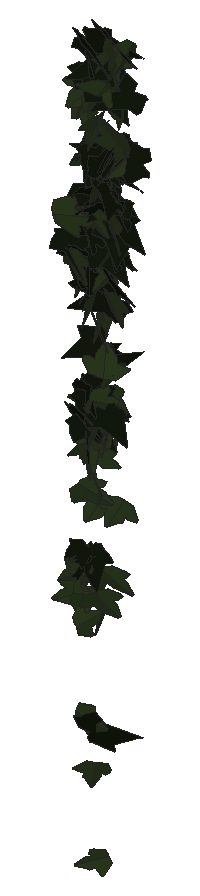
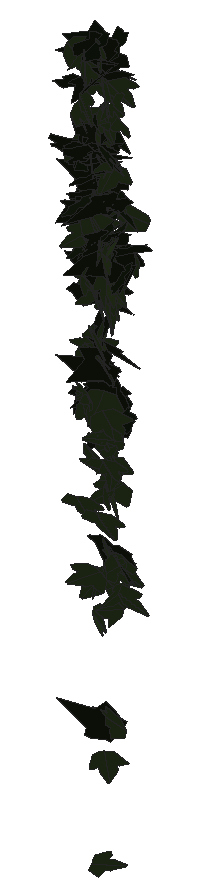
# SketchUp Ruby script. Lengths in inches.
U = 1.inch
M = Sketchup.active_model
def pt(a) = Geom::Point3d.new(a.map { |v| v * U })
def face(e, loops, mat)
  f = e.add_face(loops[0].map { |a| pt(a) })
  loops[1..].each { |l| e.add_face(l.map { |a| pt(a) }).erase! }
  f.material = f.back_material = mat if mat
  f
end
# faces: each face lists its corners as indices into pts; further lists are holes
def faces(e, pts, list, mat = nil) = list.each { |f| face(e, (f[0].is_a?(Array) ? f : [f]).map { |l| l.map { |i| pts[i] } }, mat) }
# xy, xz, yz: faces in a plane at the given z, y or x. An outline is a flat list of corners, or four numbers for a rectangle; further outlines are holes
def ring(l) = l.size == 4 ? [[l[0], l[1]], [l[2], l[1]], [l[2], l[3]], [l[0], l[3]]] : l.each_slice(2).to_a
def flat(e, list, mat, &to3) = list.each { |f| face(e, (f[0].is_a?(Array) ? f : [f]).map { |l| ring(l).map { |u, v| to3.(u, v) } }, mat) }
def xy(e, z, list, mat = nil) = flat(e, list, mat) { |x, y| [x, y, z] }
def xz(e, y, list, mat = nil) = flat(e, list, mat) { |x, z| [x, y, z] }
def yz(e, x, list, mat = nil) = flat(e, list, mat) { |y, z| [x, y, z] }
def lines(e, pts, list) = list.each { |a, b| e.add_line(pt(pts[a]), pt(pts[b])) }
# prism: a flat outline (further loops are holes) pulled along v
def prism(e, loops, v, mat = nil)
  f = face(e, loops, mat); d = Geom::Vector3d.new(v.map { |x| x * U })
  f.pushpull(f.normal.samedirection?(d) ? d.length : -d.length)
end
def box(e, o, s, mat = nil) = prism(e, [[o, [o[0] + s[0], o[1], o[2]], [o[0] + s[0], o[1] + s[1], o[2]], [o[0], o[1] + s[1], o[2]]]], [0, 0, s[2]], mat)
def at(x, y, z, deg = 0) = Geom::Transformation.translation(pt([x, y, z])) * Geom::Transformation.rotation(ORIGIN, Z_AXIS, deg.degrees)
def axes(o, x, y, z) = Geom::Transformation.new([*x, 0, *y, 0, *z, 0, *pt(o).to_a, 1])
def part(name) = M.definitions.add(name)
# library, detail: a bought-in or finely detailed component or shape, given as its bounding box
def library(name, o, s) = part(name).tap { |d| box(d.entities, o, s) }
def detail(e, o, s) = box(e.add_group.entities, o, s)
def put(e, d, t, mat = nil) = e.add_instance(d, t).tap { |i| i.material = mat if mat }
def group(e, t, mat = nil) = e.add_group.tap { |g| g.transformation = t; g.material = mat if mat }.entities
root = M.entities
M.materials.add("1026 AP 7946 SUNNY SIDE UP").color = [254, 231, 186]
M.materials.add("efeu1").color = [18, 25, 13]
M.materials.add("efeu2").color = [43, 57, 29]
c1 = part("ivyleaf_10")
p = [[0,0.5,-0.03],[-0.0625,2.02,-0.43],[-0.19,2.01,-0.46],[-0.54,1.05,-0.29],[-0.52,0.625,-0.18],[-0.83,0.76,-0.28],
  [-1.16,0.64,-0.33],[-1.15,0.33,-0.24],[-0.77,-0.39,0.02],[-0.3,-0.51,0.16],[0.04,-0.48,0.23],[-0.02,2.01,-0.4375],
  [-0.06,2.01,-0.43],[0.04,-0.49,0.23],[0.67,-0.49,0.14],[1.38,0.36,-0.2],[1.375,0.51,-0.24],[0.81,0.65,-0.19],
  [0.62,0.59,-0.15],[0.6,1.09,-0.28],[0.5,1.23,-0.31]]
faces(c1.entities,p,[[0,1,2,3,4,5,6,7,8,9,10],[11,12,0,13,14,15,16,17,18,19,20]],"efeu2")
c2 = part("ivyleaf_9")
p = [[1.54,2.16,1.25],[1.36,2.04,1.19],[-0.21,0.99,0.68],[-0.71,1.11,0.82],[-0.85,0.86,0.67],[-0.8,0.17,0.21],
  [-0.9,-0.01,0.1],[-0.67,-0.16,-0.02],[-0.08,-0.08,-0.05],[-0.03,-0.6,-0.4],[0.65,-0.88,-0.66],[0.83,-0.6,-0.49],
  [1.29,-0.42,-0.43],[1.8125,-0.07,-0.26],[1.21,0.44,0.15]]
faces(c2.entities,p,[[0,1,2,3,4,5,6,7,8,9,10,11,12,13,14]],"efeu1")
put(root,c1,axes([109.95,212.01,255.51],[0.26567,-0.027,-0.18569],[-0.28379,0.00798,-0.17561],[0.03823,0.24682,-0.01317]),"1026 AP 7946 SUNNY SIDE UP")
put(root,c1,axes([109.79,212.4,258.55],[-0.1445,-0.22327,-0.06871],[0.05185,0.05714,-0.24825],[0.36215,-0.09727,0.00812]),"1026 AP 7946 SUNNY SIDE UP")
put(root,c2,axes([109.67,212.17,263.2],[-0.09824,-0.24087,-0.06837],[0.05541,0.05781,-0.25527],[0.38836,-0.06918,0.01912]),"1026 AP 7946 SUNNY SIDE UP")
put(root,c2,axes([109.59,212.375,262.71],[0.23978,-0.1967,-0.00954],[-0.02008,0.00039,-0.2562],[0.3089,0.15271,-0.00925]),"1026 AP 7946 SUNNY SIDE UP")
put(root,c1,axes([109.92,212.48,259.55],[-0.27232,-0.15904,0.1058],[-0.08999,-0.08997,-0.24137],[0.28457,-0.18065,0.02492]),"1026 AP 7946 SUNNY SIDE UP")
put(root,c2,axes([110.05,211.97,256.21],[-0.23185,0.05497,-0.23398],[-0.32019,0.10226,0.16207],[0.18122,0.25102,-0.013]),"1026 AP 7946 SUNNY SIDE UP")
put(root,c1,axes([109.82,212.4,262.4],[0.04831,-0.21588,0.12905],[0.02946,-0.1251,-0.22537],[0.39232,0.03598,0.00103]),"1026 AP 7946 SUNNY SIDE UP")
put(root,c1,axes([109.8125,212.41,266.43],[0.06069,0.19637,-0.16477],[-0.07582,-0.15427,-0.20659],[-0.39207,0.06023,0.01445]),"1026 AP 7946 SUNNY SIDE UP")
put(root,c1,axes([109.79,212.43,264.99],[-0.22484,-0.16671,-0.10592],[0.12644,0.06482,-0.2252],[0.27997,-0.16316,0.01665]),"1026 AP 7946 SUNNY SIDE UP")
put(root,c1,axes([110.03,212.06,256],[-0.14603,-0.08892,0.19858],[-0.19182,-0.1505,-0.13261],[0.27405,-0.15273,0.01299]),"1026 AP 7946 SUNNY SIDE UP")
put(root,c1,axes([109.91,212.35,256.17],[-0.008,-0.02125,-0.24373],[-0.14537,-0.21767,0.02093],[-0.34384,0.09252,-0.00318]),"1026 AP 7946 SUNNY SIDE UP")
put(root,c1,axes([109.77,212.66,263.22],[0.07225,-0.1563,0.20212],[0.13251,-0.1792,-0.1677],[0.37266,0.09402,0.02044]),"1026 AP 7946 SUNNY SIDE UP")
put(root,c1,axes([109.89,212.4,262.07],[0.02954,-0.23161,-0.0794],[-0.00868,0.07555,-0.23895],[0.38307,0.01957,0.00071]),"1026 AP 7946 SUNNY SIDE UP")
put(root,c1,axes([109.75,211.98,262.9375],[-0.30074,0.1009,-0.14061],[0.15291,-0.10443,-0.2196],[-0.21964,-0.21086,0.03965]),"1026 AP 7946 SUNNY SIDE UP")
put(root,c1,axes([109.89,212.42,262.8],[0.0748,-0.22741,0.06651],[0.01014,-0.0659,-0.23963],[0.37213,0.04751,-0.00684]),"1026 AP 7946 SUNNY SIDE UP")
put(root,c1,axes([109.87,212.5625,258.6],[0.35432,0.03853,-0.05339],[-0.07387,-0.03241,-0.23446],[-0.07007,0.22898,-0.0228]),"1026 AP 7946 SUNNY SIDE UP")
put(root,c1,axes([109.9,212.41,261.92],[0.08031,-0.22516,-0.05453],[0.00337,0.05336,-0.23713],[0.36323,0.04929,0.01426]),"1026 AP 7946 SUNNY SIDE UP")
put(root,c1,axes([109.92,212.45,262.55],[-0.1428,-0.21605,-0.04939],[0.0373,0.04069,-0.24112],[0.34556,-0.09367,0.00562]),"1026 AP 7946 SUNNY SIDE UP")
put(root,c2,axes([109.74,212.48,263.5625],[0.05723,-0.22738,0.07709],[0.01454,-0.07561,-0.23765],[0.37676,0.03746,-0.00254]),"1026 AP 7946 SUNNY SIDE UP")
put(root,c2,axes([109.99,212.51,265.51],[-0.27707,0.09995,-0.14583],[0.16719,-0.09806,-0.20743],[-0.21608,-0.20404,0.0265]),"1026 AP 7946 SUNNY SIDE UP")
put(root,c2,axes([109.96,212.08,263.05],[0.25538,0.17305,-0.1346],[-0.11712,-0.11009,-0.2444],[-0.3212,0.17773,-0.0179]),"1026 AP 7946 SUNNY SIDE UP")
put(root,c1,axes([109.55,211.97,263.8],[0.12252,-0.05437,-0.28763],[0.44547,-0.00726,0.08296],[-0.03418,-0.28948,0.05019]),"1026 AP 7946 SUNNY SIDE UP")
put(root,c2,axes([109.74,212.375,263.54],[0.18545,-0.22028,-0.02972],[-0.03743,0.01852,-0.25699],[0.34706,0.1197,-0.01184]),"1026 AP 7946 SUNNY SIDE UP")
put(root,c1,axes([109.97,212.33,257.85],[0.1444,-0.22256,-0.03055],[-0.03458,0.0216,-0.2476],[0.35109,0.09367,-0.01183]),"1026 AP 7946 SUNNY SIDE UP")
put(root,c1,axes([109.77,212.59,263.25],[-0.11548,-0.02043,0.23444],[0.24922,-0.17689,0.03528],[0.25904,0.16108,0.07058]),"1026 AP 7946 SUNNY SIDE UP")
put(root,c1,axes([109.95,212.47,266.76],[0.19355,-0.20355,-0.09751],[-0.018,0.10083,-0.24108],[0.35176,0.11716,0.04132]),"1026 AP 7946 SUNNY SIDE UP")
put(root,c1,axes([109.74,212.35,266.08],[0.2976,-0.06782,0.16008],[0.22734,-0.05818,-0.2074],[0.1403,0.23812,-0.00349]),"1026 AP 7946 SUNNY SIDE UP")
put(root,c2,axes([109.79,212.54,263.625],[-0.02058,-0.18249,-0.18617],[0.07224,0.17532,-0.18586],[0.39616,-0.04145,0.02422]),"1026 AP 7946 SUNNY SIDE UP")
put(root,c1,axes([110.12,212.37,258.73],[0.27238,-0.00991,0.16281],[-0.24412,0.03587,0.17778],[-0.04942,-0.23177,0.01916]),"1026 AP 7946 SUNNY SIDE UP")
put(root,c2,axes([110.14,212.05,264.23],[-0.20037,0.20832,-0.07484],[0.03974,-0.07092,-0.25152],[-0.34524,-0.12906,0.01448]),"1026 AP 7946 SUNNY SIDE UP")
put(root,c2,axes([109.8125,212.39,258.73],[0.00691,-0.02381,-0.26251],[0.34379,-0.13185,0.01582],[-0.20875,-0.21793,0.01736]),"1026 AP 7946 SUNNY SIDE UP")
put(root,c1,axes([110.01,212.53,257.375],[0.39026,0.00091,-0.06405],[-0.09709,-0.02679,-0.25446],[-0.01162,0.25446,-0.02505]),"1026 AP 7946 SUNNY SIDE UP")
put(root,c2,axes([109.79,212,259.51],[0.36886,-0.08874,-0.01531],[-0.03361,-0.01609,-0.25742],[0.1373,0.23447,-0.02188]),"1026 AP 7946 SUNNY SIDE UP")
put(root,c2,axes([109.79,212.4,264.33],[0.14742,-0.1036,-0.27684],[-0.00668,0.28151,-0.11193],[0.45195,0.03795,0.08865]),"1026 AP 7946 SUNNY SIDE UP")
put(root,c2,axes([110.18,212.19,262.28],[0.14266,0.00378,0.24335],[-0.35375,0.07853,0.08819],[-0.11326,-0.24052,0.03107]),"1026 AP 7946 SUNNY SIDE UP")
put(root,c1,axes([109.74,212.43,259.1],[0.05744,0.01411,0.2255],[0.28034,0.12722,-0.03837],[-0.2007,0.18174,0.01094]),"1026 AP 7946 SUNNY SIDE UP")
put(root,c1,axes([110.08,212.18,266.75],[0.41118,0.04904,-0.14126],[-0.2038,-0.05135,-0.27331],[-0.10529,0.2909,-0.02263]),"1026 AP 7946 SUNNY SIDE UP")
put(root,c1,axes([110.12,212.5625,263.81],[-0.25043,-0.14346,0.1096],[-0.09999,-0.08882,-0.22029],[0.26326,-0.17021,0.02059]),"1026 AP 7946 SUNNY SIDE UP")
put(root,c1,axes([110.04,212.17,265.08],[0.20856,-0.18089,-0.14076],[-0.03698,0.14533,-0.22256],[0.35355,0.12191,0.05975]),"1026 AP 7946 SUNNY SIDE UP")
put(root,c1,axes([109.92,211.94,255.53],[-0.00863,-0.11387,-0.23916],[0.16901,0.20949,-0.10756],[0.36878,-0.09868,0.04369]),"1026 AP 7946 SUNNY SIDE UP")
put(root,c1,axes([110.21,212.19,257.81],[-0.10336,0.10587,-0.25616],[-0.19576,0.21597,0.12959],[0.37815,0.14074,-0.00293]),"1026 AP 7946 SUNNY SIDE UP")
put(root,c2,axes([109.82,212.47,263.83],[0.26612,-0.17408,-0.01227],[-0.01697,0.00474,-0.25005],[0.27374,0.16953,-0.00357]),"1026 AP 7946 SUNNY SIDE UP")
put(root,c1,axes([110.02,212.48,263.43],[0.10858,-0.19099,-0.14006],[0.0323,0.14504,-0.19991],[0.36623,0.04383,0.05916]),"1026 AP 7946 SUNNY SIDE UP")
put(root,c2,axes([110.23,212.31,261.04],[-0.38561,0.02596,0.03116],[-0.05095,-0.02161,-0.2529],[-0.0362,-0.24613,0.02402]),"1026 AP 7946 SUNNY SIDE UP")
put(root,c1,axes([109.98,212.26,258.51],[0.02522,0.22637,-0.07191],[-0.01019,-0.07081,-0.2342],[-0.37295,0.01724,0.00153]),"1026 AP 7946 SUNNY SIDE UP")
put(root,c2,axes([109.96,212.55,263.53],[-0.09495,-0.18649,0.14625],[-0.01104,-0.14617,-0.20026],[0.36938,-0.05231,0.03161]),"1026 AP 7946 SUNNY SIDE UP")
put(root,c1,axes([110.19,212.5,263.48],[-0.31336,-0.00999,0.12456],[-0.16673,-0.09883,-0.18896],[0.09287,-0.21114,0.08104]),"1026 AP 7946 SUNNY SIDE UP")
put(root,c2,axes([109.8,212.28,267.63],[0.22083,-0.20421,0.07857],[0.04988,-0.072,-0.25534],[0.33977,0.1433,-0.01358]),"1026 AP 7946 SUNNY SIDE UP")
put(root,c1,axes([109.95,212.36,262.16],[-0.27246,0.11802,-0.11162],[0.12287,-0.07819,-0.21561],[-0.22074,-0.1892,0.01775]),"1026 AP 7946 SUNNY SIDE UP")
put(root,c2,axes([110.07,212.44,265.26],[-0.32709,-0.00918,-0.13072],[0.19953,-0.03098,-0.21227],[-0.01316,-0.24166,0.03074]),"1026 AP 7946 SUNNY SIDE UP")
put(root,c2,axes([109.84,212.16,260.04],[-0.03416,-0.05723,-0.24539],[0.38283,-0.02853,-0.016],[-0.03782,-0.23715,0.05965]),"1026 AP 7946 SUNNY SIDE UP")
put(root,c1,axes([110.04,212.49,265.6875],[0.05156,-0.1748,0.17807],[0.07521,-0.16753,-0.18381],[0.38027,0.05684,0.01221]),"1026 AP 7946 SUNNY SIDE UP")
put(root,c2,axes([109.95,212.19,259.3],[0.01277,-0.157,-0.23612],[-0.01359,0.22815,-0.16061],[0.43547,0.01172,0.00191]),"1026 AP 7946 SUNNY SIDE UP")
put(root,c1,axes([109.86,212.01,256.2],[0.23544,0.05247,0.16186],[0.2397,0.03816,-0.16289],[-0.10073,0.21344,-0.0093]),"1026 AP 7946 SUNNY SIDE UP")
put(root,c1,axes([110.06,212.27,261.95],[0.12021,-0.22502,0.15697],[0.07674,-0.14569,-0.24568],[0.42151,0.0907,-0.00004]),"1026 AP 7946 SUNNY SIDE UP")
put(root,c1,axes([110.13,212.59,261.34],[0.20857,-0.18887,-0.02988],[-0.04371,0.01454,-0.23722],[0.29701,0.13477,-0.01393]),"1026 AP 7946 SUNNY SIDE UP")
put(root,c2,axes([109.83,212.46,263.01],[0.39086,0.03781,0.09334],[0.14651,-0.01495,-0.25761],[-0.04767,0.26408,-0.02637]),"1026 AP 7946 SUNNY SIDE UP")
put(root,c1,axes([110.03,212.38,260.39],[0.34948,-0.09622,0.00819],[0.00412,0.02733,0.24821],[-0.15183,-0.22074,0.0256]),"1026 AP 7946 SUNNY SIDE UP")
put(root,c2,axes([110.03,212.16,262.3],[-0.0398,0.00741,0.27138],[0.26926,0.20156,0.01229],[-0.31488,0.17142,-0.02379]),"1026 AP 7946 SUNNY SIDE UP")
put(root,c1,axes([110.14,212.24,265.98],[-0.01093,-0.26636,0.02833],[0.00023,-0.02903,-0.27466],[0.4213,-0.0069,0.00089]),"1026 AP 7946 SUNNY SIDE UP")
put(root,c1,axes([110.14,212.53,262.21],[0.16965,-0.2135,-0.01814],[-0.02198,0.0113,-0.24625],[0.33597,0.10855,-0.00695]),"1026 AP 7946 SUNNY SIDE UP")
put(root,c2,axes([109.96,212.4,260.69],[0.25356,0.14535,0.1393],[0.18415,0.0697,-0.22202],[-0.25095,0.19801,-0.02217]),"1026 AP 7946 SUNNY SIDE UP")
put(root,c2,axes([110.34,212.47,267.16],[-0.35792,-0.06332,0.11072],[-0.15155,-0.05387,-0.24249],[0.12529,-0.24605,0.023]),"1026 AP 7946 SUNNY SIDE UP")
put(root,c2,axes([109.83,212.41,267.6],[0.11239,0.02609,-0.27258],[0.22228,0.2285,0.06385],[0.35435,-0.15161,0.0464]),"1026 AP 7946 SUNNY SIDE UP")
put(root,c2,axes([109.98,212.57,267.04],[0.11693,-0.24067,-0.05574],[-0.03625,0.04805,-0.2591],[0.3857,0.07748,-0.00745]),"1026 AP 7946 SUNNY SIDE UP")
put(root,c2,axes([110.19,212.03,264.625],[0.08586,0.23727,0.00918],[0.01001,0.0063,-0.25074],[-0.37314,0.05477,-0.00461]),"1026 AP 7946 SUNNY SIDE UP")
put(root,c1,axes([110.03,212.51,261.28],[0.02963,-0.03524,0.2414],[0.181,-0.20434,-0.04236],[0.32604,0.11664,0.00158]),"1026 AP 7946 SUNNY SIDE UP")
put(root,c1,axes([110.27,212.27,249.58],[0.08195,0.02913,-0.22315],[-0.23509,-0.1579,-0.05981],[-0.25102,0.15739,-0.01683]),"1026 AP 7946 SUNNY SIDE UP")
put(root,c1,axes([109.97,212.09,257.82],[-0.19901,-0.12352,-0.2011],[0.27812,0.09013,-0.17701],[0.23218,-0.21384,0.03967]),"1026 AP 7946 SUNNY SIDE UP")
put(root,c1,axes([110.0625,212.08,256.12],[0.18279,-0.21681,-0.01269],[0.02773,-0.0031,0.25301],[-0.34024,-0.11674,0.0138]),"1026 AP 7946 SUNNY SIDE UP")
put(root,c1,axes([109.89,212.16,252.68],[-0.00277,-0.01772,-0.26253],[0.32415,-0.15042,0.00843],[-0.23694,-0.20559,0.0146]),"1026 AP 7946 SUNNY SIDE UP")
put(root,c1,axes([110.15,212.32,259.84],[-0.26637,-0.18507,-0.10021],[0.1161,0.06272,-0.25784],[0.30674,-0.18445,0.01057]),"1026 AP 7946 SUNNY SIDE UP")
put(root,c2,axes([109.96,212.32,267.04],[-0.00389,-0.18092,-0.21006],[0.14,0.19116,-0.17562],[0.40385,-0.06801,0.05886]),"1026 AP 7946 SUNNY SIDE UP")
put(root,c1,axes([110.48,212.27,263.68],[-0.21199,0.0051,-0.23274],[-0.34105,0.07102,0.13539],[0.09987,0.25335,-0.03167]),"1026 AP 7946 SUNNY SIDE UP")
put(root,c2,axes([110.31,212.11,265.83],[-0.22213,0.17158,-0.17272],[0.13784,-0.1454,-0.22891],[-0.35227,-0.16508,0.01934]),"1026 AP 7946 SUNNY SIDE UP")
put(root,c1,axes([110.24,212.58,267.22],[-0.04311,-0.2249,0.16696],[0.02476,-0.16513,-0.23246],[0.43635,-0.01285,0.02969]),"1026 AP 7946 SUNNY SIDE UP")
put(root,c2,axes([110.34,212.23,261.12],[0.02462,-0.1724,0.21561],[-0.03295,0.20923,0.17955],[-0.42628,-0.02613,-0.00143]),"1026 AP 7946 SUNNY SIDE UP")
put(root,c2,axes([110.17,212.71,264.84],[-0.13806,-0.22959,0.02697],[-0.0032,-0.02863,-0.25325],[0.36356,-0.08744,0.00801]),"1026 AP 7946 SUNNY SIDE UP")
put(root,c1,axes([110.33,212.21,266.75],[-0.21237,-0.203,0.14874],[-0.07681,-0.14079,-0.24983],[0.38517,-0.14,0.0322]),"1026 AP 7946 SUNNY SIDE UP")
put(root,c2,axes([110.52,212.64,265.12],[-0.20236,0.00498,0.24536],[-0.36477,-0.06402,-0.12815],[0.08495,-0.26301,0.03421]),"1026 AP 7946 SUNNY SIDE UP")
put(root,c2,axes([110.08,212.27,265.29],[0.08734,-0.21189,-0.15592],[-0.02388,0.15063,-0.2239],[0.40765,0.05422,0.02029]),"1026 AP 7946 SUNNY SIDE UP")
put(root,c2,axes([110.11,212.0625,256.5],[-0.25464,-0.09039,-0.19974],[0.29419,0.05673,-0.18841],[0.16157,-0.24576,0.02826]),"1026 AP 7946 SUNNY SIDE UP")
put(root,c1,axes([110.14,211.79,254.97],[0.08101,0.04357,-0.25588],[0.16483,0.22714,0.06472],[0.36105,-0.11348,0.02787]),"1026 AP 7946 SUNNY SIDE UP")
put(root,c2,axes([110.31,212.49,265.03],[-0.2873,-0.1676,0.05018],[-0.03924,-0.04609,-0.25511],[0.27204,-0.18365,0.01619]),"1026 AP 7946 SUNNY SIDE UP")
put(root,c1,axes([110.1,212.03,264],[-0.30628,0.02435,-0.14409],[0.21156,-0.04487,-0.20114],[-0.07193,-0.23565,0.02197]),"1026 AP 7946 SUNNY SIDE UP")
put(root,c1,axes([110.23,212.1875,259.24],[0.06699,-0.1845,0.11842],[0.05048,-0.11159,-0.19565],[0.33895,0.05309,0.00573]),"1026 AP 7946 SUNNY SIDE UP")
put(root,c1,axes([110.25,212.43,267.63],[0.2844,-0.17791,-0.05857],[-0.02007,0.06581,-0.25817],[0.29252,0.17749,0.03924]),"1026 AP 7946 SUNNY SIDE UP")
put(root,c1,axes([110.28,212.41,264.49],[0.23891,-0.19293,-0.01996],[-0.02953,0.00846,-0.25275],[0.30328,0.1528,-0.00889]),"1026 AP 7946 SUNNY SIDE UP")
put(root,c1,axes([110.31,212.01,251.76],[-0.2358,-0.17653,0.02394],[-0.00169,-0.03078,-0.238],[0.28018,-0.14876,0.01871]),"1026 AP 7946 SUNNY SIDE UP")
put(root,c1,axes([110.09,212.43,258.39],[0.31784,-0.06842,-0.09881],[0.15302,-0.00906,0.21876],[-0.10356,-0.22339,0.01996]),"1026 AP 7946 SUNNY SIDE UP")
put(root,c1,axes([110.23,212.37,255.03],[0.14268,-0.17438,0.12516],[0.07406,-0.11342,-0.20296],[0.32678,0.10184,-0.00865]),"1026 AP 7946 SUNNY SIDE UP")
put(root,c1,axes([110.27,212.25,264.39],[-0.35991,0.07393,-0.02431],[0.02629,-0.02611,-0.24712],[-0.11936,-0.22866,0.01887]),"1026 AP 7946 SUNNY SIDE UP")
put(root,c1,axes([110.4,212.45,263.72],[0.20412,-0.19123,-0.14522],[-0.15052,0.10357,-0.23678],[0.34079,0.16029,-0.0176]),"1026 AP 7946 SUNNY SIDE UP")
put(root,c2,axes([110.18,212.27,263.53],[0.14173,-0.18604,-0.18423],[-0.12338,0.15952,-0.21203],[0.38534,0.1195,-0.00013]),"1026 AP 7946 SUNNY SIDE UP")
put(root,c1,axes([110.24,212.37,262.07],[0.19121,0.19849,-0.138],[0.07648,0.12792,0.23949],[0.36969,-0.12912,0.02183]),"1026 AP 7946 SUNNY SIDE UP")
put(root,c2,axes([110.54,212.28,262.12],[0.00331,-0.00934,-0.26526],[-0.24892,-0.20314,0.00507],[-0.31954,0.15814,-0.0067]),"1026 AP 7946 SUNNY SIDE UP")
put(root,c1,axes([110.25,212.6875,262.59],[0.00726,-0.17673,0.1746],[0.10143,-0.16365,-0.17753],[0.37256,0.048,0.04493]),"1026 AP 7946 SUNNY SIDE UP")
put(root,c2,axes([110.26,212.64,265.47],[-0.25107,-0.18792,-0.06317],[0.0913,0.02934,-0.25261],[0.29657,-0.16812,0.02429]),"1026 AP 7946 SUNNY SIDE UP")
put(root,c2,axes([110.51,211.99,260.51],[-0.29664,0.06026,-0.14455],[-0.19473,0.07104,0.20288],[0.14134,0.22434,-0.02388]),"1026 AP 7946 SUNNY SIDE UP")
put(root,c1,axes([110.29,212.1,264.66],[-0.0016,-0.17066,-0.20517],[0.05977,0.19599,-0.17292],[0.40689,-0.02946,0.02459]),"1026 AP 7946 SUNNY SIDE UP")
put(root,c2,axes([110.11,212.11,259.97],[0.02142,-0.09566,-0.24752],[0.08387,0.23591,-0.09248],[0.39708,-0.04467,0.03288]),"1026 AP 7946 SUNNY SIDE UP")
put(root,c1,axes([110.35,212.36,265.11],[0.07081,-0.21164,-0.11685],[-0.02022,0.11189,-0.22205],[0.37614,0.04586,0.01006]),"1026 AP 7946 SUNNY SIDE UP")
put(root,c2,axes([110.18,212.2,265.02],[-0.0346,0.23017,0.14455],[0.02719,-0.13797,0.23737],[0.42193,0.02777,-0.00344]),"1026 AP 7946 SUNNY SIDE UP")
put(root,c1,axes([110.23,212.38,259.09],[0.22628,-0.12902,0.17567],[0.17482,-0.13145,-0.19904],[0.28828,0.18099,-0.01718]),"1026 AP 7946 SUNNY SIDE UP")
put(root,c2,axes([110.0625,212.57,267.68],[0.22291,-0.15956,0.16818],[0.15409,-0.13221,-0.22034],[0.32532,0.17195,-0.01087]),"1026 AP 7946 SUNNY SIDE UP")
put(root,c2,axes([110.5,212.1,264.25],[0.0344,0.20179,-0.13587],[-0.02701,-0.13194,-0.20986],[-0.37909,0.02771,0.00262]),"1026 AP 7946 SUNNY SIDE UP")
put(root,c2,axes([110.2,212.38,260.4375],[0.00972,0.01256,0.25009],[0.36123,0.07885,-0.00977],[-0.12459,0.22961,-0.00882]),"1026 AP 7946 SUNNY SIDE UP")
put(root,c2,axes([110.52,212.46,264.26],[-0.30023,-0.13775,0.07436],[-0.06898,-0.06322,-0.24161],[0.2352,-0.19438,0.02406]),"1026 AP 7946 SUNNY SIDE UP")
put(root,c2,axes([110.27,212.32,266.82],[-0.00882,-0.22205,-0.18428],[0.02699,0.17706,-0.22756],[0.44629,-0.0151,0.01012]),"1026 AP 7946 SUNNY SIDE UP")
put(root,c1,axes([110.49,212.28,259.51],[-0.19267,-0.18732,0.04861],[-0.02435,-0.04743,-0.2305],[0.30318,-0.12285,0.01238]),"1026 AP 7946 SUNNY SIDE UP")
put(root,c1,axes([110.46,212.4,267.21],[0.07911,-0.23001,-0.12472],[-0.00209,0.12176,-0.24079],[0.40776,0.04525,0.02297]),"1026 AP 7946 SUNNY SIDE UP")
put(root,c1,axes([110.46,212.28,262.68],[-0.0589,-0.13771,0.18537],[0.00908,-0.18367,-0.14404],[0.35715,-0.01804,0.03423]),"1026 AP 7946 SUNNY SIDE UP")
put(root,c2,axes([110.4,212.09,264.95],[-0.12279,-0.07631,0.23673],[0.26024,0.16003,0.11342],[-0.27878,0.183,0.00161]),"1026 AP 7946 SUNNY SIDE UP")
put(root,c1,axes([110.48,211.95,255.68],[-0.06529,0.14539,0.17359],[-0.11364,0.15243,-0.15371],[-0.32995,-0.08127,0.01859]),"1026 AP 7946 SUNNY SIDE UP")
put(root,c2,axes([110.13,212.57,264.78],[0.1872,-0.12129,0.18941],[0.21488,-0.12423,-0.17566],[0.27277,0.1811,0.00839]),"1026 AP 7946 SUNNY SIDE UP")
put(root,c1,axes([110.57,212.38,266.3],[0.18408,-0.11182,-0.20795],[-0.15859,0.17801,-0.16132],[0.32537,0.15002,0.03902]),"1026 AP 7946 SUNNY SIDE UP")
put(root,c1,axes([110.51,212.18,263.2],[0.10746,-0.27566,-0.04637],[-0.03425,0.03932,-0.29211],[0.43746,0.07079,-0.01148]),"1026 AP 7946 SUNNY SIDE UP")
put(root,c2,axes([110.21,212.53,265.49],[0.05001,-0.13077,0.21861],[0.17236,-0.1856,-0.13538],[0.35311,0.10912,0.03512]),"1026 AP 7946 SUNNY SIDE UP")
put(root,c1,axes([110.32,211.99,259.9],[-0.06694,-0.0927,-0.25486],[0.23578,0.19718,-0.10177],[0.34107,-0.1545,0.02033]),"1026 AP 7946 SUNNY SIDE UP")
put(root,c1,axes([110.7,212.2,265.63],[-0.34056,0.04605,-0.16351],[-0.23254,0.06374,0.22695],[0.11687,0.261,-0.02491]),"1026 AP 7946 SUNNY SIDE UP")
put(root,c1,axes([110.36,212.48,263.47],[-0.1983,-0.11526,-0.19164],[0.25252,0.09601,-0.17349],[0.23246,-0.20261,0.02497]),"1026 AP 7946 SUNNY SIDE UP")
put(root,c1,axes([110.46,212.49,267.33],[0.03774,0.24154,-0.09487],[-0.00395,-0.09364,-0.25052],[-0.40722,0.0233,-0.00636]),"1026 AP 7946 SUNNY SIDE UP")
put(root,c2,axes([110.51,212.1,264.91],[0.09614,0.12044,0.22415],[0.09923,0.20849,-0.13638],[-0.37727,0.08553,0.02125]),"1026 AP 7946 SUNNY SIDE UP")
put(root,c1,axes([110.35,212.34,255.92],[-0.26203,-0.02579,-0.17251],[0.26537,-0.00697,-0.17211],[0.0208,-0.23604,0.02254]),"1026 AP 7946 SUNNY SIDE UP")
put(root,c1,axes([110.6,212.22,260.64],[-0.13059,-0.21973,0.06728],[-0.02548,-0.06499,-0.24225],[0.3601,-0.08429,0.00726]),"1026 AP 7946 SUNNY SIDE UP")
put(root,c2,axes([110.2,212.05,252.47],[0.09718,0.00282,0.27871],[0.38887,-0.1131,-0.05765],[0.17247,0.25341,-0.02706]),"1026 AP 7946 SUNNY SIDE UP")
put(root,c1,axes([110.58,212.42,257.48],[0.36617,0.02147,-0.05925],[-0.0869,-0.02607,-0.24017],[-0.04247,0.23848,-0.0195]),"1026 AP 7946 SUNNY SIDE UP")
put(root,c1,axes([110.48,211.91,255.64],[-0.28506,-0.14189,-0.14266],[0.19014,0.0682,-0.23605],[0.24594,-0.21718,0.01714]),"1026 AP 7946 SUNNY SIDE UP")
put(root,c2,axes([110.47,212.58,263.05],[-0.07046,-0.16853,0.17839],[0.02216,-0.17859,-0.17538],[0.38039,-0.02081,0.04326]),"1026 AP 7946 SUNNY SIDE UP")
put(root,c1,axes([110.38,212.5,259.81],[-0.06806,0.00673,-0.23672],[0.22002,-0.18479,-0.03381],[-0.28686,-0.14333,0.03023]),"1026 AP 7946 SUNNY SIDE UP")
put(root,c1,axes([110.58,212.6875,267.52],[-0.04133,-0.20289,0.17634],[0.0614,-0.17423,-0.20621],[0.41404,0.00559,0.04818]),"1026 AP 7946 SUNNY SIDE UP")
put(root,c2,axes([110.43,212.6875,264.08],[0.00773,-0.20986,0.13299],[0.05536,-0.12838,-0.21516],[0.38444,0.02271,0.02831]),"1026 AP 7946 SUNNY SIDE UP")
put(root,c2,axes([110.45,212.12,263.24],[0.00639,-0.18704,-0.16323],[0.0423,0.15679,-0.19033],[0.38203,-0.01423,0.0238]),"1026 AP 7946 SUNNY SIDE UP")
put(root,c2,axes([110.79,212.55,266.68],[-0.32786,-0.11023,0.11014],[-0.1303,-0.07226,-0.24225],[0.20409,-0.2232,0.02227]),"1026 AP 7946 SUNNY SIDE UP")
put(root,c1,axes([110.59,211.93,260.6875],[0.33829,0.14757,-0.041],[0.0253,0.0479,0.26726],[0.23935,-0.21364,0.0297]),"1026 AP 7946 SUNNY SIDE UP")
put(root,c2,axes([110.51,212.2,264.54],[-0.01797,-0.21183,0.16034],[0.00378,-0.15706,-0.21928],[0.41443,-0.00775,0.00895]),"1026 AP 7946 SUNNY SIDE UP")
put(root,c2,axes([110.51,212.0625,259.71],[-0.08791,-0.15471,-0.18294],[0.10458,0.16378,-0.16844],[0.35417,-0.08676,0.00433]),"1026 AP 7946 SUNNY SIDE UP")
put(root,c2,axes([110.36,212.25,262.55],[0.18004,-0.13906,0.19445],[0.1589,-0.16124,-0.1857],[0.33375,0.15178,-0.01649]),"1026 AP 7946 SUNNY SIDE UP")
put(root,c1,axes([110.61,212.14,262.22],[-0.33568,0.136,-0.072],[0.07489,-0.05629,-0.26019],[-0.22906,-0.21771,0.02045]),"1026 AP 7946 SUNNY SIDE UP")
put(root,c2,axes([110.45,212.35,263.87],[-0.06688,-0.11268,-0.23157],[0.23678,0.17037,-0.11667],[0.3155,-0.15174,0.03847]),"1026 AP 7946 SUNNY SIDE UP")
put(root,c2,axes([110.59,212.34,263.65],[-0.11197,-0.24233,-0.01216],[0.01616,0.00785,-0.26004],[0.38105,-0.07154,0.00746]),"1026 AP 7946 SUNNY SIDE UP")
put(root,c2,axes([111.01,212.5,265.18],[-0.31932,0.04778,0.18299],[-0.28063,0.01117,-0.21357],[-0.06828,-0.26939,0.02197]),"1026 AP 7946 SUNNY SIDE UP")
put(root,c1,axes([110.72,212.14,263.4375],[-0.25781,0.18546,0.00084],[0.01872,0.01084,0.25454],[0.29102,0.1636,-0.01563]),"1026 AP 7946 SUNNY SIDE UP")
put(root,c1,axes([110.73,212.45,265.21],[0.09582,0.11056,-0.22935],[-0.12696,-0.20867,-0.13039],[-0.3706,0.10007,-0.01463]),"1026 AP 7946 SUNNY SIDE UP")
